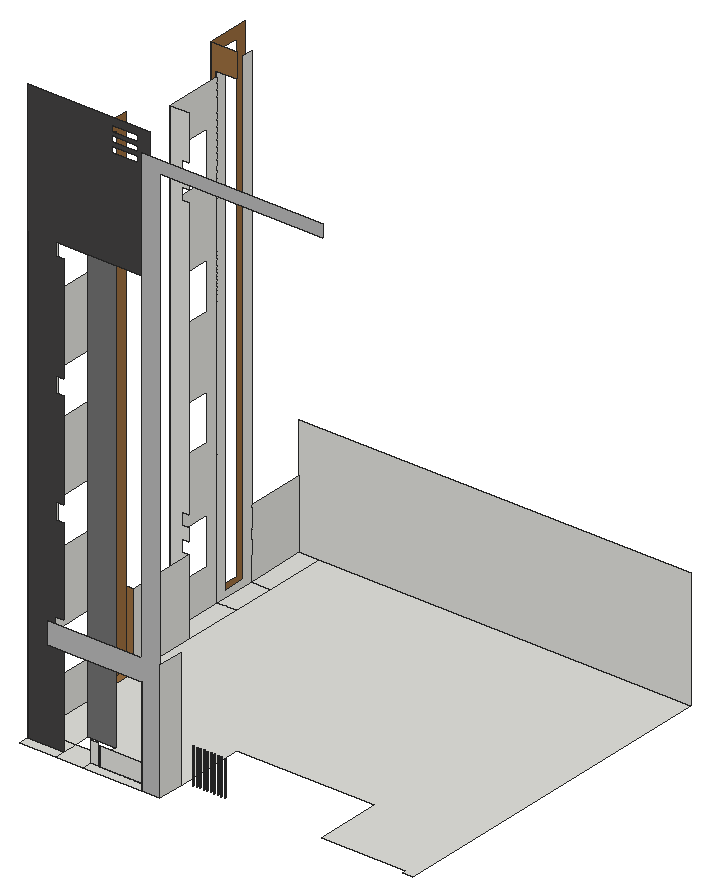
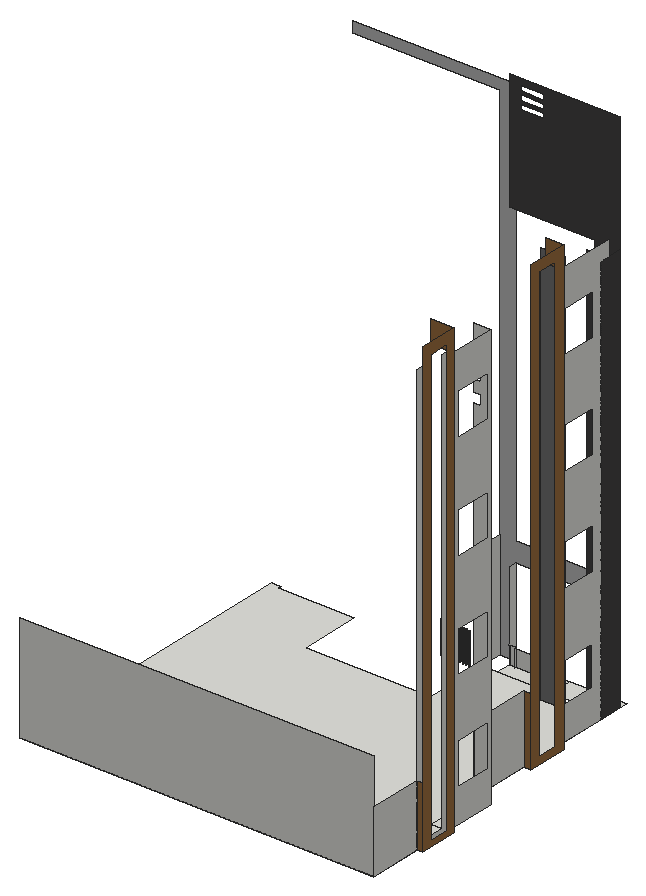
# SketchUp Ruby script. Lengths in inches.
U = 1.inch
M = Sketchup.active_model
def pt(a) = Geom::Point3d.new(a.map { |v| v * U })
def face(e, loops, mat)
  f = e.add_face(loops[0].map { |a| pt(a) })
  loops[1..].each { |l| e.add_face(l.map { |a| pt(a) }).erase! }
  f.material = f.back_material = mat if mat
  f
end
# faces: each face lists its corners as indices into pts; further lists are holes
def faces(e, pts, list, mat = nil) = list.each { |f| face(e, (f[0].is_a?(Array) ? f : [f]).map { |l| l.map { |i| pts[i] } }, mat) }
# xy, xz, yz: faces in a plane at the given z, y or x. An outline is a flat list of corners, or four numbers for a rectangle; further outlines are holes
def ring(l) = l.size == 4 ? [[l[0], l[1]], [l[2], l[1]], [l[2], l[3]], [l[0], l[3]]] : l.each_slice(2).to_a
def flat(e, list, mat, &to3) = list.each { |f| face(e, (f[0].is_a?(Array) ? f : [f]).map { |l| ring(l).map { |u, v| to3.(u, v) } }, mat) }
def xy(e, z, list, mat = nil) = flat(e, list, mat) { |x, y| [x, y, z] }
def xz(e, y, list, mat = nil) = flat(e, list, mat) { |x, z| [x, y, z] }
def yz(e, x, list, mat = nil) = flat(e, list, mat) { |y, z| [x, y, z] }
def lines(e, pts, list) = list.each { |a, b| e.add_line(pt(pts[a]), pt(pts[b])) }
# prism: a flat outline (further loops are holes) pulled along v
def prism(e, loops, v, mat = nil)
  f = face(e, loops, mat); d = Geom::Vector3d.new(v.map { |x| x * U })
  f.pushpull(f.normal.samedirection?(d) ? d.length : -d.length)
end
def box(e, o, s, mat = nil) = prism(e, [[o, [o[0] + s[0], o[1], o[2]], [o[0] + s[0], o[1] + s[1], o[2]], [o[0], o[1] + s[1], o[2]]]], [0, 0, s[2]], mat)
def at(x, y, z, deg = 0) = Geom::Transformation.translation(pt([x, y, z])) * Geom::Transformation.rotation(ORIGIN, Z_AXIS, deg.degrees)
def axes(o, x, y, z) = Geom::Transformation.new([*x, 0, *y, 0, *z, 0, *pt(o).to_a, 1])
def part(name) = M.definitions.add(name)
# library, detail: a bought-in or finely detailed component or shape, given as its bounding box
def library(name, o, s) = part(name).tap { |d| box(d.entities, o, s) }
def detail(e, o, s) = box(e.add_group.entities, o, s)
def put(e, d, t, mat = nil) = e.add_instance(d, t).tap { |i| i.material = mat if mat }
def group(e, t, mat = nil) = e.add_group.tap { |g| g.transformation = t; g.material = mat if mat }.entities
root = M.entities
M.materials.add("Generic").color = [155, 110, 63]
M.materials.add("Generic\#2").color = [186, 186, 186]
M.materials.add("[Color M05]").color = [114, 114, 114]
M.materials.add("[Granite Dark Gray]").color = [68, 67, 67]
xy(root,204.9375,[[48.5,81.125,110.7,97.25],[110.7,81.125,157.47,124.5],[157.47,81.125,259.3125,81.125,259.3125,97.25,248.28,97.25,248.28,98.375,247.78,98.375,247.78,97.25,173.03,97.25,173.03,98,172.53,98,172.53,97.25,157.47,97.25],[48.5,97.25,110.7,124.5],[157.47,97.25,157.47,124.5,259.3125,124.5,259.3125,97.25,248.28,97.25,248.28,98.375,247.78,98.375,247.78,97.25,173.03,97.25,173.03,98,172.53,98,172.53,97.25],
  [[48.5,124.5,48.5,724.5,690.4375,724.5,690.4375,124.5,673.48,124.5,673.48,130.75,528.75,130.75,528.75,246,290.4375,246,290.4375,124.5,157.47,124.5,157.47,150.6875,110.7,150.6875,110.7,124.5],[286.27,135.31,286.48,135.34,286.67,135.42,286.84,135.55,286.97,135.72,287.05,135.91,287.08,136.12,287.05,136.33,286.97,136.53,286.84,136.7,286.67,136.83,286.48,136.91,286.27,136.93,286.06,136.91,285.86,136.83,285.69,136.7,285.5625,136.53,285.48,136.33,285.45,136.12,285.48,135.91,285.5625,135.72,285.69,135.55,285.86,135.42,286.06,135.34],[280.27,135.31,280.48,135.34,280.67,135.42,280.84,135.55,280.97,135.72,281.05,135.91,281.08,136.12,281.05,136.33,280.97,136.53,280.84,136.7,280.67,136.83,280.48,136.91,280.27,136.93,280.06,136.91,279.86,136.83,279.69,136.7,279.5625,136.53,279.48,136.33,279.45,136.12,279.48,135.91,279.5625,135.72,279.69,135.55,279.86,135.42,280.06,135.34]],[15.3125,446.1875,48.5,547.73],[15.3125,547.73,48.5,619.73],[15.3125,619.73,48.5,724.5]])
xy(root,204.9375,[[35,249,48.5,326.1875],[4.375,547.73,15.3125,621.86]],"Generic")
xz(root,81.125,[[259.3125,204.9375,290.4375,204.9375,290.4375,1168.125,570.42,1168.125,570.42,1189.3125,259.3125,1189.3125,259.3125,409.46,96.41,409.46,96.41,372.9375,259.3125,372.9375]],"Generic\#2")
xz(root,97.25,[[157.47,204.9375,172.53,204.9375,172.53,236.625,170.35,236.625,170.35,239.9375,157.47,239.9375],[173.03,204.9375,247.78,236.625],[248.28,204.9375,259.3125,204.9375,259.3125,239.9375,249.19,239.9375,249.19,236.625,248.28,236.625]])
xz(root,97.25,[[[48.5,204.9375,110.7,204.9375,110.7,372.9375,96.41,372.9375,96.41,409.46,110.7,409.46,110.7,558.95,96.98,558.95,96.98,587.54,110.7,587.54,110.7,754.57,96.98,754.57,96.98,781.48,110.7,781.48,110.7,966.17,96.98,966.17,96.98,987.75,259.3125,987.75,259.3125,1214.9375,48.5,1214.9375],[193.63,1160.4,238.32,1171.15],[193.63,1176.21,238.32,1186.96],[193.63,1192.02,238.32,1202.77]]],"[Granite Dark Gray]")
xz(root,98,[[172.53,204.9375,173.03,236.625]])
xz(root,98.375,[[247.78,204.9375,248.28,236.625]])
xz(root,150.6875,[[110.7,204.9375,157.47,976.6875]],"[Color M05]")
xz(root,249,[[35,204.9375,48.5,204.9375,48.5,1016.8125,41,1016.8125,41,1024.6875,69,1024.6875,69,1067.5625,35,1067.5625]],"Generic")
xz(root,326.1875,[[35,204.9375,48.5,334.69]],"Generic")
xz(root,446.1875,[[15.3125,204.9375,48.5,204.9375,48.5,334.69,35,334.69,35,354.7,48.5,354.7,48.5,376.31,35,376.31,35,396.32,48.5,396.32,48.5,878.88,35,878.88,35,898.89,48.5,898.89,48.5,920.5,35,920.5,35,940.51,48.5,940.51,48.5,1016.8125,15.3125,1016.8125]])
xz(root,547.73,[[4.375,204.9375,15.3125,204.9375,15.3125,1016.8125,10.5,1016.8125,10.5,1024.6875,48.5,1024.6875,48.5,1067.5625,4.375,1067.5625]],"Generic")
xz(root,621.86,[[4.375,204.9375,15.3125,323.59]],"Generic")
xz(root,724.5,[[15.3125,204.9375,690.4375,409.875]])
yz(root,4.375,[[[547.73,204.9375,621.86,1067.5625],[563.94,216.21,603.53,1046.8125]]],"Generic")
yz(root,15.3125,[[[446.1875,204.9375,547.73,1016.8125],[454.08,866.77,525.8,946],[454.08,663.96,525.8,743.18],[454.08,461.15,525.8,540.37],[454.08,270.33,525.8,349.56]],[547.73,204.9375,621.86,204.9375,621.86,1024.6875,603.53,1024.6875,603.53,216.21,563.94,216.21,563.94,1024.6875,547.73,1024.6875],[621.86,204.9375,724.5,323.59]])
yz(root,35,[[[249,204.9375,326.1875,1067.5625],[268.32,219.07,306.87,1046.8125]]],"Generic")
yz(root,48.5,[[[143.77,204.9375,143.77,987.75,124.5,987.75,124.5,1016.8125,249,1016.8125,249,204.9375],[161.95,866.52,234.18,946.25],[161.95,666.77,234.18,746.5],[161.95,467.02,234.18,546.75],[164.2,269.52,231.93,344.75]],[326.1875,204.9375,446.1875,334.69]])
yz(root,48.5,[[97.25,204.9375,143.77,987.75]],"[Granite Dark Gray]")
yz(root,172.53,[[97.25,204.9375,98,236.625]])
yz(root,173.03,[[97.25,204.9375,98,236.625]])
yz(root,247.78,[[97.25,204.9375,98.375,236.625]])
yz(root,248.28,[[97.25,204.9375,98.375,236.625]])
yz(root,259.3125,[[81.125,204.9375,81.125,372.9375,97.25,372.9375,97.25,240.4375,98.375,240.4375,98.375,239.9375,97.25,239.9375,97.25,204.9375]])
yz(root,290.4375,[[81.125,204.9375,124.5,409.875]])
p = [[303.49,135.42,204.9375],[303.68,135.34,204.9375],[303.68,135.34,264.83],[303.49,135.42,264.83],[303.89,135.31,204.9375],[303.89,135.31,264.83],
  [304.1,135.34,204.9375],[304.1,135.34,264.83],[304.3,135.42,204.9375],[304.3,135.42,264.83],[309.86,135.42,204.9375],[310.06,135.34,204.9375],
  [310.06,135.34,264.83],[309.86,135.42,264.83],[310.27,135.31,204.9375],[310.27,135.31,264.83],[310.48,135.34,204.9375],[310.48,135.34,264.83],
  [310.67,135.42,204.9375],[310.67,135.42,264.83],[315.86,135.42,204.9375],[316.06,135.34,204.9375],[316.06,135.34,264.83],[315.86,135.42,264.83],
  [316.27,135.31,204.9375],[316.27,135.31,264.83],[316.48,135.34,204.9375],[316.48,135.34,264.83],[316.67,135.42,204.9375],[316.67,135.42,264.83],
  [321.86,135.42,204.9375],[322.06,135.34,204.9375],[322.06,135.34,264.83],[321.86,135.42,264.83],[322.27,135.31,204.9375],[322.27,135.31,264.83],
  [322.48,135.34,204.9375],[322.48,135.34,264.83],[322.67,135.42,204.9375],[322.67,135.42,264.83],[327.86,135.42,204.9375],[328.06,135.34,204.9375],
  [328.06,135.34,264.83],[327.86,135.42,264.83],[328.27,135.31,204.9375],[328.27,135.31,264.83],[328.48,135.34,204.9375],[328.48,135.34,264.83],
  [328.67,135.42,204.9375],[328.67,135.42,264.83],[333.86,135.42,204.9375],[334.06,135.34,204.9375],[334.06,135.34,264.83],[333.86,135.42,264.83],
  [334.27,135.31,204.9375],[334.27,135.31,264.83],[334.48,135.34,204.9375],[334.48,135.34,264.83],[334.67,135.42,204.9375],[334.67,135.42,264.83],
  [339.86,135.42,204.9375],[340.06,135.34,204.9375],[340.06,135.34,264.83],[339.86,135.42,264.83],[340.27,135.31,204.9375],[340.27,135.31,264.83],
  [340.48,135.34,204.9375],[340.48,135.34,264.83],[340.67,135.42,204.9375],[340.67,135.42,264.83],[345.86,135.42,204.9375],[346.06,135.34,204.9375],
  [346.06,135.34,264.83],[345.86,135.42,264.83],[346.27,135.31,204.9375],[346.27,135.31,264.83],[346.48,135.34,204.9375],[346.48,135.34,264.83],
  [346.67,135.42,204.9375],[346.67,135.42,264.83],[351.86,135.42,204.9375],[352.06,135.34,204.9375],[352.06,135.34,264.83],[351.86,135.42,264.83],
  [352.27,135.31,204.9375],[352.27,135.31,264.83],[352.48,135.34,204.9375],[352.48,135.34,264.83],[352.67,135.42,204.9375],[352.67,135.42,264.83],
  [357.86,135.42,204.9375],[358.06,135.34,204.9375],[358.06,135.34,264.83],[357.86,135.42,264.83],[358.27,135.31,204.9375],[358.27,135.31,264.83],
  [358.48,135.34,204.9375],[358.48,135.34,264.83],[358.67,135.42,204.9375],[358.67,135.42,264.83],[303.32,135.55,204.9375],[303.32,135.55,264.83],
  [304.47,135.55,204.9375],[304.47,135.55,264.83],[309.69,135.55,204.9375],[309.69,135.55,264.83],[310.84,135.55,204.9375],[310.84,135.55,264.83],
  [315.69,135.55,204.9375],[315.69,135.55,264.83],[316.84,135.55,204.9375],[316.84,135.55,264.83],[321.69,135.55,204.9375],[321.69,135.55,264.83],
  [322.84,135.55,204.9375],[322.84,135.55,264.83],[327.69,135.55,204.9375],[327.69,135.55,264.83],[328.84,135.55,204.9375],[328.84,135.55,264.83],
  [333.69,135.55,204.9375],[333.69,135.55,264.83],[334.84,135.55,204.9375],[334.84,135.55,264.83],[339.69,135.55,204.9375],[339.69,135.55,264.83],
  [340.84,135.55,204.9375],[340.84,135.55,264.83],[345.69,135.55,204.9375],[345.69,135.55,264.83],[346.84,135.55,204.9375],[346.84,135.55,264.83],
  [351.69,135.55,204.9375],[351.69,135.55,264.83],[352.84,135.55,204.9375],[352.84,135.55,264.83],[357.69,135.55,204.9375],[357.69,135.55,264.83],
  [358.84,135.55,204.9375],[358.84,135.55,264.83],[303.1875,135.72,204.9375],[303.1875,135.72,264.83],[304.6,135.72,204.9375],[304.6,135.72,264.83],
  [309.5625,135.72,204.9375],[309.5625,135.72,264.83],[310.97,135.72,204.9375],[310.97,135.72,264.83],[315.5625,135.72,204.9375],[315.5625,135.72,264.83],
  [316.97,135.72,204.9375],[316.97,135.72,264.83],[321.5625,135.72,204.9375],[321.5625,135.72,264.83],[322.97,135.72,204.9375],[322.97,135.72,264.83],
  [327.5625,135.72,204.9375],[327.5625,135.72,264.83],[328.97,135.72,204.9375],[328.97,135.72,264.83],[333.5625,135.72,204.9375],[333.5625,135.72,264.83],
  [334.97,135.72,204.9375],[334.97,135.72,264.83],[339.5625,135.72,204.9375],[339.5625,135.72,264.83],[340.97,135.72,204.9375],[340.97,135.72,264.83],
  [345.5625,135.72,204.9375],[345.5625,135.72,264.83],[346.97,135.72,204.9375],[346.97,135.72,264.83],[351.5625,135.72,204.9375],[351.5625,135.72,264.83],
  [352.97,135.72,204.9375],[352.97,135.72,264.83],[357.5625,135.72,204.9375],[357.5625,135.72,264.83],[303.11,135.91,204.9375],[303.11,135.91,264.83],
  [304.68,135.91,204.9375],[304.68,135.91,264.83],[309.48,135.91,204.9375],[309.48,135.91,264.83],[311.05,135.91,204.9375],[311.05,135.91,264.83],
  [315.48,135.91,204.9375],[315.48,135.91,264.83],[317.05,135.91,204.9375],[317.05,135.91,264.83],[321.48,135.91,204.9375],[321.48,135.91,264.83],
  [323.05,135.91,204.9375],[323.05,135.91,264.83],[327.48,135.91,204.9375],[327.48,135.91,264.83],[329.05,135.91,204.9375],[329.05,135.91,264.83],
  [333.48,135.91,204.9375],[333.48,135.91,264.83],[335.05,135.91,204.9375],[335.05,135.91,264.83],[339.48,135.91,204.9375],[339.48,135.91,264.83],
  [341.05,135.91,204.9375],[341.05,135.91,264.83],[345.48,135.91,204.9375],[345.48,135.91,264.83],[347.05,135.91,204.9375],[347.05,135.91,264.83],
  [351.48,135.91,204.9375],[351.48,135.91,264.83],[353.05,135.91,204.9375],[353.05,135.91,264.83],[357.48,135.91,204.9375],[357.48,135.91,264.83],
  [303.08,136.12,204.9375],[303.08,136.12,264.83],[304.7,136.12,204.9375],[304.7,136.12,264.83],[309.45,136.12,204.9375],[309.45,136.12,264.83],
  [311.08,136.12,204.9375],[311.08,136.12,264.83],[315.45,136.12,204.9375],[315.45,136.12,264.83],[317.08,136.12,204.9375],[317.08,136.12,264.83],
  [321.45,136.12,204.9375],[321.45,136.12,264.83],[323.08,136.12,204.9375],[323.08,136.12,264.83],[327.45,136.12,204.9375],[327.45,136.12,264.83],
  [329.08,136.12,204.9375],[329.08,136.12,264.83],[333.45,136.12,204.9375],[333.45,136.12,264.83],[335.08,136.12,204.9375],[335.08,136.12,264.83],
  [339.45,136.12,204.9375],[339.45,136.12,264.83],[341.08,136.12,204.9375],[341.08,136.12,264.83],[345.45,136.12,204.9375],[345.45,136.12,264.83],
  [347.08,136.12,204.9375],[347.08,136.12,264.83],[351.45,136.12,204.9375],[351.45,136.12,264.83],[353.08,136.12,204.9375],[353.08,136.12,264.83],
  [357.45,136.12,204.9375],[357.45,136.12,264.83],[303.11,136.33,204.9375],[303.11,136.33,264.83],[304.68,136.33,204.9375],[304.68,136.33,264.83],
  [309.48,136.33,204.9375],[309.48,136.33,264.83],[311.05,136.33,204.9375],[311.05,136.33,264.83],[315.48,136.33,204.9375],[315.48,136.33,264.83],
  [317.05,136.33,204.9375],[317.05,136.33,264.83],[321.48,136.33,204.9375],[321.48,136.33,264.83],[323.05,136.33,204.9375],[323.05,136.33,264.83],
  [327.48,136.33,204.9375],[327.48,136.33,264.83],[329.05,136.33,204.9375],[329.05,136.33,264.83],[333.48,136.33,204.9375],[333.48,136.33,264.83],
  [335.05,136.33,204.9375],[335.05,136.33,264.83],[339.48,136.33,204.9375],[339.48,136.33,264.83],[341.05,136.33,204.9375],[341.05,136.33,264.83],
  [345.48,136.33,204.9375],[345.48,136.33,264.83],[347.05,136.33,204.9375],[347.05,136.33,264.83],[351.48,136.33,204.9375],[351.48,136.33,264.83],
  [353.05,136.33,204.9375],[353.05,136.33,264.83],[357.48,136.33,204.9375],[357.48,136.33,264.83],[303.1875,136.53,204.9375],[303.1875,136.53,264.83],
  [304.6,136.53,204.9375],[304.6,136.53,264.83],[309.5625,136.53,204.9375],[309.5625,136.53,264.83],[310.97,136.53,204.9375],[310.97,136.53,264.83],
  [315.5625,136.53,204.9375],[315.5625,136.53,264.83],[316.97,136.53,204.9375],[316.97,136.53,264.83],[321.5625,136.53,204.9375],[321.5625,136.53,264.83],
  [322.97,136.53,204.9375],[322.97,136.53,264.83],[327.5625,136.53,204.9375],[327.5625,136.53,264.83],[328.97,136.53,204.9375],[328.97,136.53,264.83],
  [333.5625,136.53,204.9375],[333.5625,136.53,264.83],[334.97,136.53,204.9375],[334.97,136.53,264.83],[339.5625,136.53,204.9375],[339.5625,136.53,264.83],
  [340.97,136.53,204.9375],[340.97,136.53,264.83],[345.5625,136.53,204.9375],[345.5625,136.53,264.83],[346.97,136.53,204.9375],[346.97,136.53,264.83],
  [351.5625,136.53,204.9375],[351.5625,136.53,264.83],[352.97,136.53,204.9375],[352.97,136.53,264.83],[357.5625,136.53,204.9375],[357.5625,136.53,264.83],
  [303.32,136.7,204.9375],[303.32,136.7,264.83],[304.47,136.7,204.9375],[304.47,136.7,264.83],[309.69,136.7,204.9375],[309.69,136.7,264.83],
  [310.84,136.7,204.9375],[310.84,136.7,264.83],[315.69,136.7,204.9375],[315.69,136.7,264.83],[316.84,136.7,204.9375],[316.84,136.7,264.83],
  [321.69,136.7,204.9375],[321.69,136.7,264.83],[322.84,136.7,204.9375],[322.84,136.7,264.83],[327.69,136.7,204.9375],[327.69,136.7,264.83],
  [328.84,136.7,204.9375],[328.84,136.7,264.83],[333.69,136.7,204.9375],[333.69,136.7,264.83],[334.84,136.7,204.9375],[334.84,136.7,264.83],
  [339.69,136.7,204.9375],[339.69,136.7,264.83],[340.84,136.7,204.9375],[340.84,136.7,264.83],[345.69,136.7,204.9375],[345.69,136.7,264.83],
  [346.84,136.7,204.9375],[346.84,136.7,264.83],[351.69,136.7,204.9375],[351.69,136.7,264.83],[352.84,136.7,204.9375],[352.84,136.7,264.83],
  [357.69,136.7,204.9375],[357.69,136.7,264.83],[358.97,136.53,204.9375],[358.84,136.7,204.9375],[358.84,136.7,264.83],[358.97,136.53,264.83],
  [303.49,136.83,204.9375],[303.49,136.83,264.83],[304.3,136.83,204.9375],[304.3,136.83,264.83],[309.86,136.83,204.9375],[309.86,136.83,264.83],
  [310.67,136.83,204.9375],[310.67,136.83,264.83],[315.86,136.83,204.9375],[315.86,136.83,264.83],[316.67,136.83,204.9375],[316.67,136.83,264.83],
  [321.86,136.83,204.9375],[321.86,136.83,264.83],[322.67,136.83,204.9375],[322.67,136.83,264.83],[327.86,136.83,204.9375],[327.86,136.83,264.83],
  [328.67,136.83,204.9375],[328.67,136.83,264.83],[333.86,136.83,204.9375],[333.86,136.83,264.83],[334.67,136.83,204.9375],[334.67,136.83,264.83],
  [339.86,136.83,204.9375],[339.86,136.83,264.83],[340.67,136.83,204.9375],[340.67,136.83,264.83],[345.86,136.83,204.9375],[345.86,136.83,264.83],
  [346.67,136.83,204.9375],[346.67,136.83,264.83],[351.86,136.83,204.9375],[351.86,136.83,264.83],[352.67,136.83,204.9375],[352.67,136.83,264.83],
  [357.86,136.83,204.9375],[357.86,136.83,264.83],[358.67,136.83,204.9375],[358.67,136.83,264.83],[303.68,136.91,204.9375],[303.68,136.91,264.83],
  [304.1,136.91,204.9375],[304.1,136.91,264.83],[310.06,136.91,204.9375],[310.06,136.91,264.83],[310.48,136.91,204.9375],[310.48,136.91,264.83],
  [316.06,136.91,204.9375],[316.06,136.91,264.83],[316.48,136.91,204.9375],[316.48,136.91,264.83],[322.06,136.91,204.9375],[322.06,136.91,264.83],
  [322.48,136.91,204.9375],[322.48,136.91,264.83],[328.06,136.91,204.9375],[328.06,136.91,264.83],[328.48,136.91,204.9375],[328.48,136.91,264.83],
  [334.06,136.91,204.9375],[334.06,136.91,264.83],[334.48,136.91,204.9375],[334.48,136.91,264.83],[340.06,136.91,204.9375],[340.06,136.91,264.83],
  [340.48,136.91,204.9375],[340.48,136.91,264.83],[346.06,136.91,204.9375],[346.06,136.91,264.83],[346.48,136.91,204.9375],[346.48,136.91,264.83],
  [352.06,136.91,204.9375],[352.06,136.91,264.83],[352.48,136.91,204.9375],[352.48,136.91,264.83],[358.06,136.91,204.9375],[358.06,136.91,264.83],
  [358.48,136.91,204.9375],[358.48,136.91,264.83],[303.89,136.93,204.9375],[303.89,136.93,264.83],[310.27,136.93,204.9375],[310.27,136.93,264.83],
  [316.27,136.93,204.9375],[316.27,136.93,264.83],[322.27,136.93,204.9375],[322.27,136.93,264.83],[328.27,136.93,204.9375],[328.27,136.93,264.83],
  [334.27,136.93,204.9375],[334.27,136.93,264.83],[340.27,136.93,204.9375],[340.27,136.93,264.83],[346.27,136.93,204.9375],[346.27,136.93,264.83],
  [352.27,136.93,204.9375],[352.27,136.93,264.83],[358.27,136.93,204.9375],[358.27,136.93,264.83]]
faces(root,p,[[0,1,2,3],[1,4,5,2],[4,6,7,5],[6,8,9,7],[10,11,12,13],[11,14,15,12],[14,16,17,15],[16,18,19,17],
  [20,21,22,23],[21,24,25,22],[24,26,27,25],[26,28,29,27],[30,31,32,33],[31,34,35,32],[34,36,37,35],[36,38,39,37],
  [40,41,42,43],[41,44,45,42],[44,46,47,45],[46,48,49,47],[50,51,52,53],[51,54,55,52],[54,56,57,55],[56,58,59,57],
  [60,61,62,63],[61,64,65,62],[64,66,67,65],[66,68,69,67],[70,71,72,73],[71,74,75,72],[74,76,77,75],[76,78,79,77],
  [80,81,82,83],[81,84,85,82],[84,86,87,85],[86,88,89,87],[90,91,92,93],[91,94,95,92],[94,96,97,95],[96,98,99,97],
  [100,0,3,101],[8,102,103,9],[104,10,13,105],[18,106,107,19],[108,20,23,109],[28,110,111,29],[112,30,33,113],[38,114,115,39],
  [116,40,43,117],[48,118,119,49],[120,50,53,121],[58,122,123,59],[124,60,63,125],[68,126,127,69],[128,70,73,129],[78,130,131,79],
  [132,80,83,133],[88,134,135,89],[136,90,93,137],[98,138,139,99],[140,100,101,141],[102,142,143,103],[144,104,105,145],[106,146,147,107],
  [148,108,109,149],[110,150,151,111],[152,112,113,153],[114,154,155,115],[156,116,117,157],[118,158,159,119],[160,120,121,161],[122,162,163,123],
  [164,124,125,165],[126,166,167,127],[168,128,129,169],[130,170,171,131],[172,132,133,173],[134,174,175,135],[176,136,137,177],[178,140,141,179],
  [142,180,181,143],[182,144,145,183],[146,184,185,147],[186,148,149,187],[150,188,189,151],[190,152,153,191],[154,192,193,155],[194,156,157,195],
  [158,196,197,159],[198,160,161,199],[162,200,201,163],[202,164,165,203],[166,204,205,167],[206,168,169,207],[170,208,209,171],[210,172,173,211],
  [174,212,213,175],[214,176,177,215],[216,178,179,217],[180,218,219,181],[220,182,183,221],[184,222,223,185],[224,186,187,225],[188,226,227,189],
  [228,190,191,229],[192,230,231,193],[232,194,195,233],[196,234,235,197],[236,198,199,237],[200,238,239,201],[240,202,203,241],[204,242,243,205],
  [244,206,207,245],[208,246,247,209],[248,210,211,249],[212,250,251,213],[252,214,215,253],[254,216,217,255],[218,256,257,219],[258,220,221,259],
  [222,260,261,223],[262,224,225,263],[226,264,265,227],[266,228,229,267],[230,268,269,231],[270,232,233,271],[234,272,273,235],[274,236,237,275],
  [238,276,277,239],[278,240,241,279],[242,280,281,243],[282,244,245,283],[246,284,285,247],[286,248,249,287],[250,288,289,251],[290,252,253,291],
  [292,254,255,293],[256,294,295,257],[296,258,259,297],[260,298,299,261],[300,262,263,301],[264,302,303,265],[304,266,267,305],[268,306,307,269],
  [308,270,271,309],[272,310,311,273],[312,274,275,313],[276,314,315,277],[316,278,279,317],[280,318,319,281],[320,282,283,321],[284,322,323,285],
  [324,286,287,325],[288,326,327,289],[328,290,291,329],[330,292,293,331],[294,332,333,295],[334,296,297,335],[298,336,337,299],[338,300,301,339],
  [302,340,341,303],[342,304,305,343],[306,344,345,307],[346,308,309,347],[310,348,349,311],[350,312,313,351],[314,352,353,315],[354,316,317,355],
  [318,356,357,319],[358,320,321,359],[322,360,361,323],[362,324,325,363],[326,364,365,327],[366,328,329,367],[368,369,370,371],[372,330,331,373],
  [332,374,375,333],[376,334,335,377],[336,378,379,337],[380,338,339,381],[340,382,383,341],[384,342,343,385],[344,386,387,345],[388,346,347,389],
  [348,390,391,349],[392,350,351,393],[352,394,395,353],[396,354,355,397],[356,398,399,357],[400,358,359,401],[360,402,403,361],[404,362,363,405],
  [364,406,407,365],[408,366,367,409],[369,410,411,370],[412,372,373,413],[374,414,415,375],[416,376,377,417],[378,418,419,379],[420,380,381,421],
  [382,422,423,383],[424,384,385,425],[386,426,427,387],[428,388,389,429],[390,430,431,391],[432,392,393,433],[394,434,435,395],[436,396,397,437],
  [398,438,439,399],[440,400,401,441],[402,442,443,403],[444,404,405,445],[406,446,447,407],[448,408,409,449],[410,450,451,411],[452,412,413,453],
  [414,452,453,415],[454,416,417,455],[418,454,455,419],[456,420,421,457],[422,456,457,423],[458,424,425,459],[426,458,459,427],[460,428,429,461],
  [430,460,461,431],[462,432,433,463],[434,462,463,435],[464,436,437,465],[438,464,465,439],[466,440,441,467],[442,466,467,443],[468,444,445,469],
  [446,468,469,447],[470,448,449,471],[450,470,471,451]])
